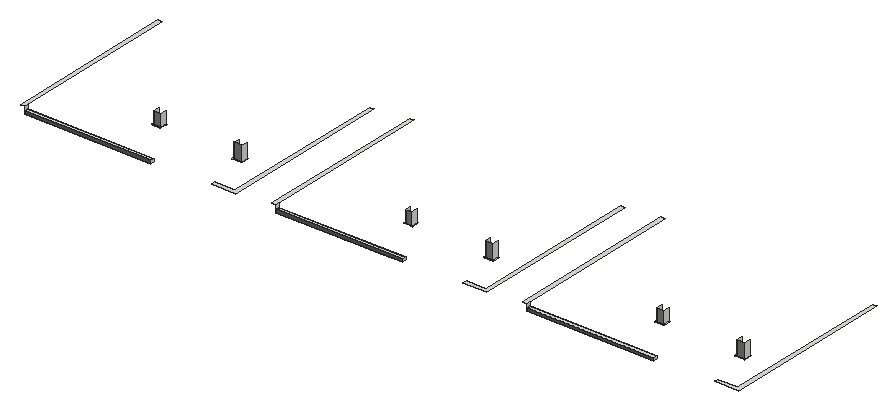
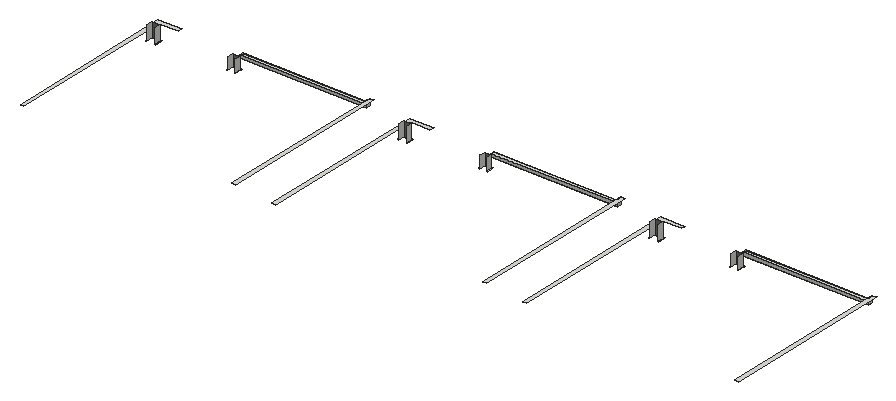
# SketchUp Ruby script. Lengths in inches.
U = 1.inch
M = Sketchup.active_model
def pt(a) = Geom::Point3d.new(a.map { |v| v * U })
def face(e, loops, mat)
  f = e.add_face(loops[0].map { |a| pt(a) })
  loops[1..].each { |l| e.add_face(l.map { |a| pt(a) }).erase! }
  f.material = f.back_material = mat if mat
  f
end
# faces: each face lists its corners as indices into pts; further lists are holes
def faces(e, pts, list, mat = nil) = list.each { |f| face(e, (f[0].is_a?(Array) ? f : [f]).map { |l| l.map { |i| pts[i] } }, mat) }
# xy, xz, yz: faces in a plane at the given z, y or x. An outline is a flat list of corners, or four numbers for a rectangle; further outlines are holes
def ring(l) = l.size == 4 ? [[l[0], l[1]], [l[2], l[1]], [l[2], l[3]], [l[0], l[3]]] : l.each_slice(2).to_a
def flat(e, list, mat, &to3) = list.each { |f| face(e, (f[0].is_a?(Array) ? f : [f]).map { |l| ring(l).map { |u, v| to3.(u, v) } }, mat) }
def xy(e, z, list, mat = nil) = flat(e, list, mat) { |x, y| [x, y, z] }
def xz(e, y, list, mat = nil) = flat(e, list, mat) { |x, z| [x, y, z] }
def yz(e, x, list, mat = nil) = flat(e, list, mat) { |y, z| [x, y, z] }
def lines(e, pts, list) = list.each { |a, b| e.add_line(pt(pts[a]), pt(pts[b])) }
# prism: a flat outline (further loops are holes) pulled along v
def prism(e, loops, v, mat = nil)
  f = face(e, loops, mat); d = Geom::Vector3d.new(v.map { |x| x * U })
  f.pushpull(f.normal.samedirection?(d) ? d.length : -d.length)
end
def box(e, o, s, mat = nil) = prism(e, [[o, [o[0] + s[0], o[1], o[2]], [o[0] + s[0], o[1] + s[1], o[2]], [o[0], o[1] + s[1], o[2]]]], [0, 0, s[2]], mat)
def at(x, y, z, deg = 0) = Geom::Transformation.translation(pt([x, y, z])) * Geom::Transformation.rotation(ORIGIN, Z_AXIS, deg.degrees)
def axes(o, x, y, z) = Geom::Transformation.new([*x, 0, *y, 0, *z, 0, *pt(o).to_a, 1])
def part(name) = M.definitions.add(name)
# library, detail: a bought-in or finely detailed component or shape, given as its bounding box
def library(name, o, s) = part(name).tap { |d| box(d.entities, o, s) }
def detail(e, o, s) = box(e.add_group.entities, o, s)
def put(e, d, t, mat = nil) = e.add_instance(d, t).tap { |i| i.material = mat if mat }
def group(e, t, mat = nil) = e.add_group.tap { |g| g.transformation = t; g.material = mat if mat }.entities
root = M.entities
M.materials.add("[Color M05]1").color = [114, 114, 114]
M.materials.add("[Color M06]1").color = [86, 86, 86]
xy(root,73.375,[[50.98,201.42,79.2,206.8],[79.2,201.42,79.2,206.8,50.98,206.8,50.98,209.86,334.6,209.86,334.6,201.42,286.58,201.42,286.58,202.49,214.81,202.49,214.81,201.42,212.66,201.42,212.66,202.49,205.65,202.49,205.65,201.42,203.17,201.42,203.17,202.49,176.08,202.49,176.08,201.42,109.22,201.42,109.22,202.49,107.42,202.49,107.42,201.42],[107.42,201.42,109.22,202.49],[176.08,201.42,203.17,202.49],[205.65,201.42,212.66,202.49],
  [214.81,201.42,286.58,202.49],[614.1,201.42,642.32,206.8],[642.32,201.42,642.32,206.8,614.1,206.8,614.1,209.86,897.73,209.86,897.73,201.42,849.71,201.42,849.71,202.49,777.93,202.49,777.93,201.42,775.78,201.42,775.78,202.49,768.78,202.49,768.78,201.42,766.29,201.42,766.29,202.49,739.2,202.49,739.2,201.42,672.34,201.42,672.34,202.49,670.54,202.49,670.54,201.42],[670.54,201.42,672.34,202.49],[739.2,201.42,766.29,202.49],
  [768.78,201.42,775.78,202.49],[777.93,201.42,849.71,202.49],[1177.23,201.42,1205.45,206.8],[1205.45,201.42,1205.45,206.8,1177.23,206.8,1177.23,209.86,1460.85,209.86,1460.85,201.42,1412.83,201.42,1412.83,202.49,1341.06,202.49,1341.06,201.42,1338.91,201.42,1338.91,202.49,1331.9,202.49,1331.9,201.42,1329.42,201.42,1329.42,202.49,1302.33,202.49,1302.33,201.42,1235.47,201.42,1235.47,202.49,1233.67,202.49,1233.67,201.42],[1233.67,201.42,1235.47,202.49],
  [1302.33,201.42,1329.42,202.49],[1331.9,201.42,1338.91,202.49],[1341.06,201.42,1412.83,202.49]])
xy(root,79.75,[[50.98,201.42,334.6,209.86],[470.8125,201.42,523.75,201.42,523.75,587.49,515.375,587.49,515.375,209.86,470.8125,209.86],[614.1,201.42,897.73,209.86],[1033.9375,201.42,1086.875,201.42,1086.875,587.49,1078.5,587.49,1078.5,209.86,1033.9375,209.86],[1177.23,201.42,1460.85,209.86],
  [1597.0625,201.42,1650,201.42,1650,587.49,1641.625,587.49,1641.625,209.86,1597.0625,209.86]])
xy(root,88.625,[[41.875,201.42,50.98,587.49],[605,201.42,614.1,587.49],[1168.125,201.42,1177.23,587.49]])
xy(root,93.74,[[456.45,275.67,458.89,278.1],[458.89,275.67,476.45,278.1],[476.45,275.67,478.89,278.1],[1019.57,275.67,1022.01,278.1],[1022.01,275.67,1039.57,278.1],
  [1039.57,275.67,1042.01,278.1],[1582.7,275.67,1585.14,278.1],[1585.14,275.67,1602.7,278.1],[1602.7,275.67,1605.14,278.1],[456.45,278.1,457.95,291.17],
  [457.95,278.1,458.89,291.17],[476.45,278.1,478.89,291.17],[1019.57,278.1,1021.07,291.17],[1021.07,278.1,1022.01,291.17],[1039.57,278.1,1042.01,291.17],
  [1582.7,278.1,1584.2,291.17],[1584.2,278.1,1585.14,291.17],[1602.7,278.1,1605.14,291.17]])
xy(root,99.34,[[277.82,275.67,280.26,278.1],[280.26,275.67,295.26,278.1],[295.26,275.67,297.7,278.1],[840.95,275.67,843.39,278.1],[843.39,275.67,858.39,278.1],
  [858.39,275.67,860.82,278.1],[1404.07,275.67,1406.51,278.1],[1406.51,275.67,1421.51,278.1],[1421.51,275.67,1423.95,278.1],[277.82,278.1,280.26,291.17],
  [295.26,278.1,297.7,291.17],[840.95,278.1,843.39,291.17],[858.39,278.1,860.82,291.17],[1404.07,278.1,1406.51,291.17],[1421.51,278.1,1423.95,291.17]])
xz(root,201.42,[[50.98,73.375,334.6,79.75],[614.1,73.375,897.73,79.75],[1177.23,73.375,1460.85,79.75]],"[Color M06]1")
xz(root,209.86,[[50.98,73.375,334.6,79.75],[614.1,73.375,897.73,79.75],[1177.23,73.375,1460.85,79.75]])
xz(root,278.1,[[458.89,93.74,476.45,126],[1022.01,93.74,1039.57,126],[1585.14,93.74,1602.7,126],[280.26,99.34,295.26,126],[843.39,99.34,858.39,126],
  [1406.51,99.34,1421.51,126]],"[Color M05]1")
yz(root,50.98,[[201.42,73.375,209.86,79.75],[201.42,79.75,209.86,88.625]])
yz(root,280.26,[[278.1,99.34,291.17,126]])
yz(root,295.26,[[278.1,99.34,291.17,126]])
yz(root,334.6,[[201.42,73.375,209.86,79.75]])
yz(root,458.89,[[278.1,93.74,291.17,126]])
yz(root,476.45,[[278.1,93.74,291.17,126]])
yz(root,614.1,[[201.42,73.375,209.86,79.75],[201.42,79.75,209.86,88.625]])
yz(root,843.39,[[278.1,99.34,291.17,126]])
yz(root,858.39,[[278.1,99.34,291.17,126]])
yz(root,897.73,[[201.42,73.375,209.86,79.75]])
yz(root,1022.01,[[278.1,93.74,291.17,126]])
yz(root,1039.57,[[278.1,93.74,291.17,126]])
yz(root,1177.23,[[201.42,73.375,209.86,79.75],[201.42,79.75,209.86,88.625]])
yz(root,1406.51,[[278.1,99.34,291.17,126]])
yz(root,1421.51,[[278.1,99.34,291.17,126]])
yz(root,1460.85,[[201.42,73.375,209.86,79.75]])
yz(root,1585.14,[[278.1,93.74,291.17,126]])
yz(root,1602.7,[[278.1,93.74,291.17,126]])
